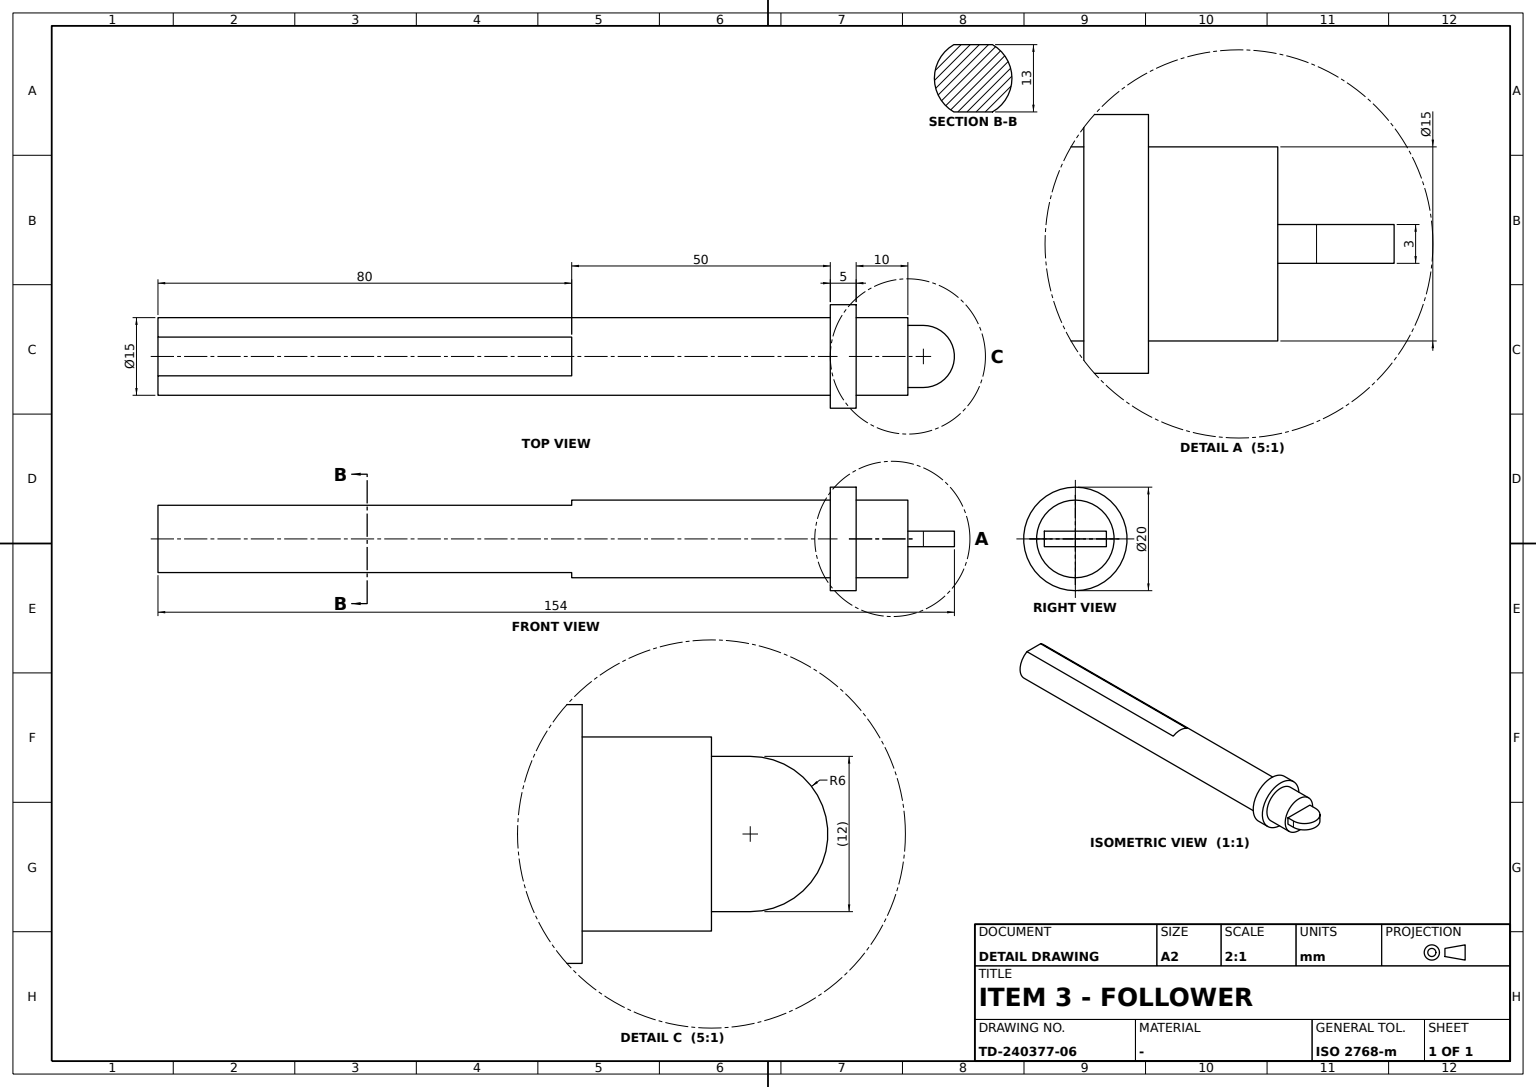
ISO-10303-21;
HEADER;
FILE_DESCRIPTION((''),'2;1');
FILE_NAME('','',(''),(''),'','','');
FILE_SCHEMA(('AUTOMOTIVE_DESIGN'));
ENDSEC;
DATA;
#1=APPLICATION_CONTEXT('');
#2=PRODUCT_CONTEXT('',#1,'mechanical');
#3=PRODUCT('','','',(#2));
#4=PRODUCT_DEFINITION_FORMATION('','',#3);
#5=PRODUCT_DEFINITION_CONTEXT('',#1,'design');
#6=PRODUCT_DEFINITION('','',#4,#5);
#7=PRODUCT_DEFINITION_SHAPE('','',#6);
#8=(LENGTH_UNIT()NAMED_UNIT(*)SI_UNIT(.MILLI.,.METRE.));
#9=(NAMED_UNIT(*)PLANE_ANGLE_UNIT()SI_UNIT($,.RADIAN.));
#10=(NAMED_UNIT(*)SI_UNIT($,.STERADIAN.)SOLID_ANGLE_UNIT());
#11=UNCERTAINTY_MEASURE_WITH_UNIT(LENGTH_MEASURE(0.005),#8,'distance_accuracy_value','');
#12=(GEOMETRIC_REPRESENTATION_CONTEXT(3)GLOBAL_UNCERTAINTY_ASSIGNED_CONTEXT((#11))GLOBAL_UNIT_ASSIGNED_CONTEXT((#8,#9,#10))REPRESENTATION_CONTEXT('',''));
#13=CARTESIAN_POINT('',(-6.5,-3.741657,80.));
#14=VERTEX_POINT('',#13);
#15=CARTESIAN_POINT('',(-6.5,3.741657,80.));
#16=VERTEX_POINT('',#15);
#17=DIRECTION('',(0.,1.,0.));
#18=VECTOR('',#17,1000.);
#19=LINE('',#13,#18);
#20=EDGE_CURVE('',#14,#16,#19,.T.);
#21=ORIENTED_EDGE('',*,*,#20,.T.);
#22=CARTESIAN_POINT('',(-6.5,3.741657,0.));
#23=VERTEX_POINT('',#22);
#24=DIRECTION('',(0.,0.,1.));
#25=VECTOR('',#24,1000.);
#26=LINE('',#22,#25);
#27=EDGE_CURVE('',#23,#16,#26,.T.);
#28=ORIENTED_EDGE('',*,*,#27,.F.);
#29=CARTESIAN_POINT('',(-6.5,-3.741657,0.));
#30=VERTEX_POINT('',#29);
#31=CARTESIAN_POINT('',(-6.5,0.,0.));
#32=LINE('',#31,#18);
#33=EDGE_CURVE('',#30,#23,#32,.T.);
#34=ORIENTED_EDGE('',*,*,#33,.F.);
#35=LINE('',#29,#25);
#36=EDGE_CURVE('',#14,#30,#35,.F.);
#37=ORIENTED_EDGE('',*,*,#36,.F.);
#38=EDGE_LOOP('',(#21,#28,#34,#37));
#39=FACE_BOUND('',#38,.T.);
#40=DIRECTION('',(1.,0.,0.));
#41=AXIS2_PLACEMENT_3D('',#29,#40,#17);
#42=PLANE('',#41);
#43=ADVANCED_FACE('',(#39),#42,.F.);
#44=CARTESIAN_POINT('',(1.5,6.,148.));
#45=VERTEX_POINT('',#44);
#46=CARTESIAN_POINT('',(1.5,6.,145.));
#47=VERTEX_POINT('',#46);
#48=CARTESIAN_POINT('',(1.5,6.,0.));
#49=DIRECTION('',(0.,0.,-1.));
#50=VECTOR('',#49,1000.);
#51=LINE('',#48,#50);
#52=EDGE_CURVE('',#45,#47,#51,.T.);
#53=ORIENTED_EDGE('',*,*,#52,.T.);
#54=CARTESIAN_POINT('',(-1.5,6.,145.));
#55=VERTEX_POINT('',#54);
#56=CARTESIAN_POINT('',(0.,6.,145.));
#57=VECTOR('',#40,1000.);
#58=LINE('',#56,#57);
#59=EDGE_CURVE('',#55,#47,#58,.T.);
#60=ORIENTED_EDGE('',*,*,#59,.F.);
#61=CARTESIAN_POINT('',(-1.5,6.,148.));
#62=VERTEX_POINT('',#61);
#63=CARTESIAN_POINT('',(-1.5,6.,0.));
#64=LINE('',#63,#50);
#65=EDGE_CURVE('',#62,#55,#64,.T.);
#66=ORIENTED_EDGE('',*,*,#65,.F.);
#67=CARTESIAN_POINT('',(0.,6.,148.));
#68=LINE('',#67,#57);
#69=EDGE_CURVE('',#62,#45,#68,.T.);
#70=ORIENTED_EDGE('',*,*,#69,.T.);
#71=EDGE_LOOP('',(#53,#60,#66,#70));
#72=FACE_BOUND('',#71,.T.);
#73=DIRECTION('',(0.,-1.,0.));
#74=AXIS2_PLACEMENT_3D('',#67,#73,#49);
#75=PLANE('',#74);
#76=ADVANCED_FACE('',(#72),#75,.F.);
#77=CARTESIAN_POINT('',(6.5,-3.741657,0.));
#78=VERTEX_POINT('',#77);
#79=CARTESIAN_POINT('',(0.,0.,0.));
#80=AXIS2_PLACEMENT_3D('',#79,#24,#40);
#81=CIRCLE('',#80,7.5);
#82=EDGE_CURVE('',#30,#78,#81,.T.);
#83=ORIENTED_EDGE('',*,*,#82,.F.);
#84=ORIENTED_EDGE('',*,*,#33,.T.);
#85=CARTESIAN_POINT('',(6.5,3.741657,0.));
#86=VERTEX_POINT('',#85);
#87=EDGE_CURVE('',#86,#23,#81,.T.);
#88=ORIENTED_EDGE('',*,*,#87,.F.);
#89=CARTESIAN_POINT('',(6.5,0.,0.));
#90=LINE('',#89,#18);
#91=EDGE_CURVE('',#78,#86,#90,.T.);
#92=ORIENTED_EDGE('',*,*,#91,.F.);
#93=EDGE_LOOP('',(#83,#84,#88,#92));
#94=FACE_BOUND('',#93,.T.);
#95=AXIS2_PLACEMENT_3D('',#79,#24,#17);
#96=PLANE('',#95);
#97=ADVANCED_FACE('',(#94),#96,.F.);
#98=CARTESIAN_POINT('',(-1.5,-6.,148.));
#99=VERTEX_POINT('',#98);
#100=CARTESIAN_POINT('',(1.5,-6.,148.));
#101=VERTEX_POINT('',#100);
#102=CARTESIAN_POINT('',(0.,-6.,148.));
#103=LINE('',#102,#57);
#104=EDGE_CURVE('',#99,#101,#103,.T.);
#105=ORIENTED_EDGE('',*,*,#104,.T.);
#106=CARTESIAN_POINT('',(1.5,0.,148.));
#107=AXIS2_PLACEMENT_3D('',#106,#40,#49);
#108=CIRCLE('',#107,6.);
#109=EDGE_CURVE('',#45,#101,#108,.T.);
#110=ORIENTED_EDGE('',*,*,#109,.F.);
#111=ORIENTED_EDGE('',*,*,#69,.F.);
#112=CARTESIAN_POINT('',(-1.5,0.,148.));
#113=AXIS2_PLACEMENT_3D('',#112,#40,#49);
#114=CIRCLE('',#113,6.);
#115=EDGE_CURVE('',#62,#99,#114,.T.);
#116=ORIENTED_EDGE('',*,*,#115,.T.);
#117=EDGE_LOOP('',(#105,#110,#111,#116));
#118=FACE_BOUND('',#117,.T.);
#119=CARTESIAN_POINT('',(0.,0.,148.));
#120=AXIS2_PLACEMENT_3D('',#119,#40,#17);
#121=CYLINDRICAL_SURFACE('',#120,6.);
#122=ADVANCED_FACE('',(#118),#121,.T.);
#123=ORIENTED_EDGE('',*,*,#65,.T.);
#124=CARTESIAN_POINT('',(-1.5,-6.,145.));
#125=VERTEX_POINT('',#124);
#126=CARTESIAN_POINT('',(-1.5,0.,145.));
#127=LINE('',#126,#18);
#128=EDGE_CURVE('',#125,#55,#127,.T.);
#129=ORIENTED_EDGE('',*,*,#128,.F.);
#130=CARTESIAN_POINT('',(-1.5,-6.,0.));
#131=LINE('',#130,#25);
#132=EDGE_CURVE('',#125,#99,#131,.T.);
#133=ORIENTED_EDGE('',*,*,#132,.T.);
#134=ORIENTED_EDGE('',*,*,#115,.F.);
#135=EDGE_LOOP('',(#123,#129,#133,#134));
#136=FACE_BOUND('',#135,.T.);
#137=CARTESIAN_POINT('',(-1.5,0.,0.));
#138=AXIS2_PLACEMENT_3D('',#137,#40,#17);
#139=PLANE('',#138);
#140=ADVANCED_FACE('',(#136),#139,.F.);
#141=CARTESIAN_POINT('',(10.,0.,130.));
#142=VERTEX_POINT('',#141);
#143=CARTESIAN_POINT('',(0.,0.,130.));
#144=AXIS2_PLACEMENT_3D('',#143,#24,#40);
#145=CIRCLE('',#144,10.);
#146=EDGE_CURVE('',#142,#142,#145,.T.);
#147=ORIENTED_EDGE('',*,*,#146,.F.);
#148=EDGE_LOOP('',(#147));
#149=FACE_BOUND('',#148,.T.);
#150=CARTESIAN_POINT('',(7.5,0.,130.));
#151=VERTEX_POINT('',#150);
#152=CIRCLE('',#144,7.5);
#153=EDGE_CURVE('',#151,#151,#152,.T.);
#154=ORIENTED_EDGE('',*,*,#153,.T.);
#155=EDGE_LOOP('',(#154));
#156=FACE_BOUND('',#155,.T.);
#157=PLANE('',#144);
#158=ADVANCED_FACE('',(#149,#156),#157,.F.);
#159=CARTESIAN_POINT('',(7.5,0.,145.));
#160=VERTEX_POINT('',#159);
#161=CARTESIAN_POINT('',(0.,0.,145.));
#162=AXIS2_PLACEMENT_3D('',#161,#24,#40);
#163=CIRCLE('',#162,7.5);
#164=EDGE_CURVE('',#160,#160,#163,.T.);
#165=ORIENTED_EDGE('',*,*,#164,.T.);
#166=EDGE_LOOP('',(#165));
#167=FACE_BOUND('',#166,.T.);
#168=ORIENTED_EDGE('',*,*,#59,.T.);
#169=CARTESIAN_POINT('',(1.5,-6.,145.));
#170=VERTEX_POINT('',#169);
#171=CARTESIAN_POINT('',(1.5,0.,145.));
#172=LINE('',#171,#18);
#173=EDGE_CURVE('',#170,#47,#172,.T.);
#174=ORIENTED_EDGE('',*,*,#173,.F.);
#175=CARTESIAN_POINT('',(0.,-6.,145.));
#176=LINE('',#175,#57);
#177=EDGE_CURVE('',#125,#170,#176,.T.);
#178=ORIENTED_EDGE('',*,*,#177,.F.);
#179=ORIENTED_EDGE('',*,*,#128,.T.);
#180=EDGE_LOOP('',(#168,#174,#178,#179));
#181=FACE_BOUND('',#180,.T.);
#182=PLANE('',#162);
#183=ADVANCED_FACE('',(#167,#181),#182,.T.);
#184=CARTESIAN_POINT('',(1.5,-6.,0.));
#185=LINE('',#184,#25);
#186=EDGE_CURVE('',#170,#101,#185,.T.);
#187=ORIENTED_EDGE('',*,*,#186,.T.);
#188=ORIENTED_EDGE('',*,*,#104,.F.);
#189=ORIENTED_EDGE('',*,*,#132,.F.);
#190=ORIENTED_EDGE('',*,*,#177,.T.);
#191=EDGE_LOOP('',(#187,#188,#189,#190));
#192=FACE_BOUND('',#191,.T.);
#193=AXIS2_PLACEMENT_3D('',#175,#17,#24);
#194=PLANE('',#193);
#195=ADVANCED_FACE('',(#192),#194,.F.);
#196=ORIENTED_EDGE('',*,*,#27,.T.);
#197=CARTESIAN_POINT('',(0.,0.,80.));
#198=DIRECTION('',(-1.,0.,0.));
#199=AXIS2_PLACEMENT_3D('',#197,#49,#198);
#200=CIRCLE('',#199,7.5);
#201=EDGE_CURVE('',#16,#14,#200,.F.);
#202=ORIENTED_EDGE('',*,*,#201,.T.);
#203=ORIENTED_EDGE('',*,*,#36,.T.);
#204=ORIENTED_EDGE('',*,*,#82,.T.);
#205=CARTESIAN_POINT('',(6.5,-3.741657,80.));
#206=VERTEX_POINT('',#205);
#207=LINE('',#77,#25);
#208=EDGE_CURVE('',#206,#78,#207,.F.);
#209=ORIENTED_EDGE('',*,*,#208,.F.);
#210=CARTESIAN_POINT('',(6.5,3.741657,80.));
#211=VERTEX_POINT('',#210);
#212=EDGE_CURVE('',#206,#211,#200,.F.);
#213=ORIENTED_EDGE('',*,*,#212,.T.);
#214=LINE('',#85,#25);
#215=EDGE_CURVE('',#86,#211,#214,.T.);
#216=ORIENTED_EDGE('',*,*,#215,.F.);
#217=ORIENTED_EDGE('',*,*,#87,.T.);
#218=EDGE_LOOP('',(#196,#202,#203,#204,#209,#213,#216,#217));
#219=FACE_BOUND('',#218,.T.);
#220=ORIENTED_EDGE('',*,*,#153,.F.);
#221=EDGE_LOOP('',(#220));
#222=FACE_BOUND('',#221,.T.);
#223=CARTESIAN_POINT('',(0.,0.,40.));
#224=AXIS2_PLACEMENT_3D('',#223,#24,#17);
#225=CYLINDRICAL_SURFACE('',#224,7.5);
#226=ADVANCED_FACE('',(#219,#222),#225,.T.);
#227=ORIENTED_EDGE('',*,*,#173,.T.);
#228=ORIENTED_EDGE('',*,*,#52,.F.);
#229=ORIENTED_EDGE('',*,*,#109,.T.);
#230=ORIENTED_EDGE('',*,*,#186,.F.);
#231=EDGE_LOOP('',(#227,#228,#229,#230));
#232=FACE_BOUND('',#231,.T.);
#233=CARTESIAN_POINT('',(1.5,0.,0.));
#234=AXIS2_PLACEMENT_3D('',#233,#40,#17);
#235=PLANE('',#234);
#236=ADVANCED_FACE('',(#232),#235,.T.);
#237=CARTESIAN_POINT('',(10.,0.,135.));
#238=VERTEX_POINT('',#237);
#239=CARTESIAN_POINT('',(0.,0.,135.));
#240=AXIS2_PLACEMENT_3D('',#239,#24,#40);
#241=CIRCLE('',#240,10.);
#242=EDGE_CURVE('',#238,#238,#241,.T.);
#243=ORIENTED_EDGE('',*,*,#242,.T.);
#244=EDGE_LOOP('',(#243));
#245=FACE_BOUND('',#244,.T.);
#246=CARTESIAN_POINT('',(7.5,0.,135.));
#247=VERTEX_POINT('',#246);
#248=CIRCLE('',#240,7.5);
#249=EDGE_CURVE('',#247,#247,#248,.T.);
#250=ORIENTED_EDGE('',*,*,#249,.F.);
#251=EDGE_LOOP('',(#250));
#252=FACE_BOUND('',#251,.T.);
#253=PLANE('',#240);
#254=ADVANCED_FACE('',(#245,#252),#253,.T.);
#255=LINE('',#205,#18);
#256=EDGE_CURVE('',#206,#211,#255,.T.);
#257=ORIENTED_EDGE('',*,*,#256,.F.);
#258=ORIENTED_EDGE('',*,*,#208,.T.);
#259=ORIENTED_EDGE('',*,*,#91,.T.);
#260=ORIENTED_EDGE('',*,*,#215,.T.);
#261=EDGE_LOOP('',(#257,#258,#259,#260));
#262=FACE_BOUND('',#261,.T.);
#263=AXIS2_PLACEMENT_3D('',#77,#40,#17);
#264=PLANE('',#263);
#265=ADVANCED_FACE('',(#262),#264,.T.);
#266=ORIENTED_EDGE('',*,*,#201,.F.);
#267=ORIENTED_EDGE('',*,*,#20,.F.);
#268=EDGE_LOOP('',(#266,#267));
#269=FACE_BOUND('',#268,.T.);
#270=AXIS2_PLACEMENT_3D('',#197,#49,#40);
#271=PLANE('',#270);
#272=ADVANCED_FACE('',(#269),#271,.T.);
#273=ORIENTED_EDGE('',*,*,#249,.T.);
#274=EDGE_LOOP('',(#273));
#275=FACE_BOUND('',#274,.T.);
#276=ORIENTED_EDGE('',*,*,#164,.F.);
#277=EDGE_LOOP('',(#276));
#278=FACE_BOUND('',#277,.T.);
#279=ADVANCED_FACE('',(#275,#278),#225,.T.);
#280=ORIENTED_EDGE('',*,*,#242,.F.);
#281=EDGE_LOOP('',(#280));
#282=FACE_BOUND('',#281,.T.);
#283=ORIENTED_EDGE('',*,*,#146,.T.);
#284=EDGE_LOOP('',(#283));
#285=FACE_BOUND('',#284,.T.);
#286=CARTESIAN_POINT('',(0.,0.,132.5));
#287=AXIS2_PLACEMENT_3D('',#286,#24,#40);
#288=CYLINDRICAL_SURFACE('',#287,10.);
#289=ADVANCED_FACE('',(#282,#285),#288,.T.);
#290=ORIENTED_EDGE('',*,*,#212,.F.);
#291=ORIENTED_EDGE('',*,*,#256,.T.);
#292=EDGE_LOOP('',(#290,#291));
#293=FACE_BOUND('',#292,.T.);
#294=ADVANCED_FACE('',(#293),#271,.T.);
#295=CLOSED_SHELL('',(#43,#76,#97,#122,#140,#158,#183,#195,#226,#236,#254,#265,#272,#279,#289,#294));
#296=MANIFOLD_SOLID_BREP('',#295);
#297=ADVANCED_BREP_SHAPE_REPRESENTATION('',(#296),#12);
#298=SHAPE_DEFINITION_REPRESENTATION(#7,#297);
ENDSEC;
END-ISO-10303-21;
